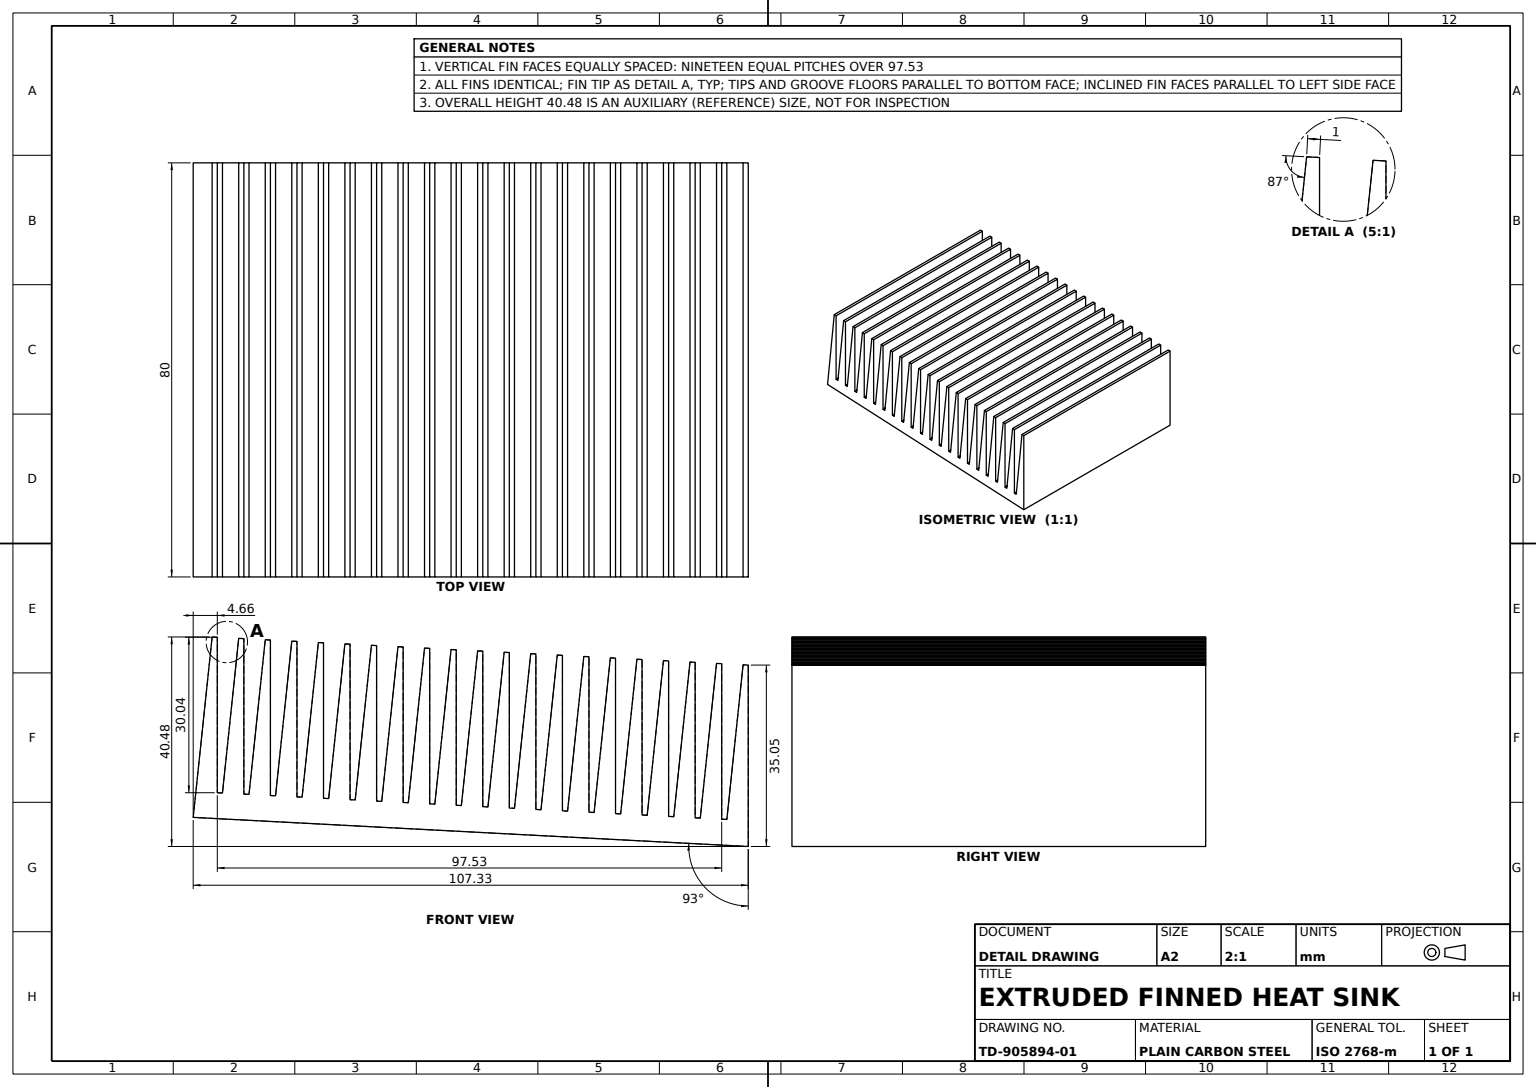
solid
v1 (-8.153019,80,-17.547966)
v2 (-6.580786,80,12.452034)
e1 v1 v2 LINE
v3 (-6.580786,0,12.452034)
e2 v2 v3 LINE
v4 (-8.153019,0,-17.547966)
e3 v4 v3 LINE
e4 v1 v4 LINE
face PLANE(AX(P(-7.213557,80,0.378046),D(0.998629535,0,-0.052335956),D(-0.052335956,0,-0.998629535))) [e1 e2 -e3 -e4]
v5 (-24.573019,80,-17.547966)
v6 (-24.573019,0,-17.547966)
e5 v5 v6 LINE
v7 (-26.145253,0,12.452034)
e6 v7 v6 LINE
v8 (-26.145253,80,12.452034)
e7 v8 v7 LINE
e8 v8 v5 LINE
face PLANE(AX(P(-25.422844,80,-1.332355),D(-0.998629535,0,-0.052335956),D(-0.052335956,0,0.998629535))) [e5 -e6 -e7 e8]
v9 (-11.720786,0,12.452034)
v10 (-10.725253,0,12.452034)
e9 v9 v10 LINE
v11 (-11.720786,80,12.452034)
e10 v11 v9 LINE
v12 (-10.725253,80,12.452034)
e11 v11 v12 LINE
e12 v12 v10 LINE
face PLANE(AX(P(0,80,12.452034),D(0,0,-1),D(-1,0,0))) [-e9 -e10 e11 e12]
v13 (1.126981,80,-17.547966)
v14 (2.126981,80,-17.547966)
e13 v13 v14 LINE
v15 (2.126981,0,-17.547966)
e14 v14 v15 LINE
v16 (1.126981,0,-17.547966)
e15 v16 v15 LINE
e16 v13 v16 LINE
face PLANE(AX(P(0,80,-17.547966),D(0,0,-1),D(-1,0,0))) [e13 e14 -e15 -e16]
v17 (-23.573019,0,-17.547966)
e17 v6 v17 LINE
v18 (-23.573019,80,-17.547966)
e18 v5 v18 LINE
e19 v18 v17 LINE
face PLANE(AX(P(0,80,-17.547966),D(0,0,-1),D(-1,0,0))) [-e17 -e5 e18 e19]
v19 (34.539214,80,12.452034)
v20 (34.539214,0,12.452034)
e20 v19 v20 LINE
v21 (32.966981,0,-17.547966)
e21 v21 v20 LINE
v22 (32.966981,80,-17.547966)
e22 v22 v21 LINE
e23 v22 v19 LINE
face PLANE(AX(P(33.793813,80,-1.771059),D(0.998629535,0,-0.052335956),D(-0.052335956,0,-0.998629535))) [e20 -e21 -e22 e23]
v23 (3.699214,80,12.452034)
v24 (3.699214,0,12.452034)
e24 v23 v24 LINE
v25 (4.694747,80,12.452034)
e25 v23 v25 LINE
v26 (4.694747,0,12.452034)
e26 v25 v26 LINE
e27 v24 v26 LINE
face PLANE(AX(P(0,80,12.452034),D(0,0,-1),D(-1,0,0))) [-e24 e25 e26 -e27]
v27 (48.386981,0,-17.547966)
v28 (49.959214,0,12.452034)
e28 v27 v28 LINE
v29 (48.386981,80,-17.547966)
e29 v29 v27 LINE
v30 (49.959214,80,12.452034)
e30 v29 v30 LINE
e31 v30 v28 LINE
face PLANE(AX(P(49.171577,80,-2.576973),D(0.998629535,0,-0.052335956),D(-0.052335956,0,-0.998629535))) [-e28 -e29 e30 e31]
v31 (50.954747,80,12.452034)
v32 (52.526981,80,-17.547966)
e32 v31 v32 LINE
v33 (52.526981,0,-17.547966)
e33 v32 v33 LINE
v34 (50.954747,0,12.452034)
e34 v34 v33 LINE
e35 v31 v34 LINE
face PLANE(AX(P(51.465975,80,2.697217),D(-0.998629535,0,-0.052335956),D(-0.052335956,0,0.998629535))) [e32 e33 -e34 -e35]
v35 (-16.860786,80,12.452034)
v36 (-15.865253,80,12.452034)
e36 v35 v36 LINE
v37 (-15.865253,0,12.452034)
e37 v36 v37 LINE
v38 (-16.860786,0,12.452034)
e38 v38 v37 LINE
e39 v35 v38 LINE
face PLANE(AX(P(0,80,12.452034),D(0,0,-1),D(-1,0,0))) [e36 e37 -e38 -e39]
v39 (40.674747,80,12.452034)
v40 (40.674747,0,12.452034)
e40 v39 v40 LINE
v41 (39.679214,0,12.452034)
e41 v41 v40 LINE
v42 (39.679214,80,12.452034)
e42 v42 v41 LINE
e43 v42 v39 LINE
face PLANE(AX(P(0,80,12.452034),D(0,0,-1),D(-1,0,0))) [e40 -e41 -e42 e43]
v43 (-5.585253,80,12.452034)
v44 (-5.585253,0,12.452034)
e44 v43 v44 LINE
e45 v3 v44 LINE
e46 v2 v43 LINE
face PLANE(AX(P(0,80,12.452034),D(0,0,-1),D(-1,0,0))) [e44 -e45 -e2 e46]
v45 (19.119214,0,12.452034)
v46 (20.114747,0,12.452034)
e47 v45 v46 LINE
v47 (19.119214,80,12.452034)
e48 v47 v45 LINE
v48 (20.114747,80,12.452034)
e49 v47 v48 LINE
e50 v48 v46 LINE
face PLANE(AX(P(0,80,12.452034),D(0,0,-1),D(-1,0,0))) [-e47 -e48 e49 e50]
v49 (8.839214,80,12.452034)
v50 (8.839214,0,12.452034)
e51 v49 v50 LINE
v51 (7.266981,0,-17.547966)
e52 v51 v50 LINE
v52 (7.266981,80,-17.547966)
e53 v52 v51 LINE
e54 v52 v49 LINE
face PLANE(AX(P(8.164207,80,-0.427868),D(0.998629535,0,-0.052335956),D(-0.052335956,0,-0.998629535))) [e51 -e52 -e53 e54]
v53 (-13.293019,80,-17.547966)
v54 (-13.293019,0,-17.547966)
e55 v53 v54 LINE
v55 (-14.293019,0,-17.547966)
e56 v55 v54 LINE
v56 (-14.293019,80,-17.547966)
e57 v56 v55 LINE
e58 v56 v53 LINE
face PLANE(AX(P(0,80,-17.547966),D(0,0,-1),D(-1,0,0))) [e55 -e56 -e57 e58]
v57 (56.094747,80,12.452034)
v58 (57.666981,80,-17.547966)
e59 v57 v58 LINE
v59 (57.666981,0,-17.547966)
e60 v58 v59 LINE
v60 (56.094747,0,12.452034)
e61 v60 v59 LINE
e62 v57 v60 LINE
face PLANE(AX(P(56.591897,80,2.965856),D(-0.998629535,0,-0.052335956),D(-0.052335956,0,0.998629535))) [e59 e60 -e61 -e62]
v61 (-32.280786,0,12.452034)
v62 (-31.285253,0,12.452034)
e63 v61 v62 LINE
v63 (-32.280786,80,12.452034)
e64 v63 v61 LINE
v64 (-31.285253,80,12.452034)
e65 v63 v64 LINE
e66 v64 v62 LINE
face PLANE(AX(P(0,80,12.452034),D(0,0,-1),D(-1,0,0))) [-e63 -e64 e65 e66]
e67 v54 v9 LINE
e68 v53 v11 LINE
face PLANE(AX(P(-12.339478,80,0.646685),D(0.998629535,0,-0.052335956),D(-0.052335956,0,-0.998629535))) [-e67 -e55 e68 e10]
v65 (53.526981,80,-17.547966)
v66 (53.526981,0,-17.547966)
e69 v65 v66 LINE
e70 v33 v66 LINE
e71 v32 v65 LINE
face PLANE(AX(P(0,80,-17.547966),D(0,0,-1),D(-1,0,0))) [e69 -e70 -e33 e71]
v67 (26.826981,80,-17.547966)
v68 (27.826981,80,-17.547966)
e72 v67 v68 LINE
v69 (27.826981,0,-17.547966)
e73 v68 v69 LINE
v70 (26.826981,0,-17.547966)
e74 v70 v69 LINE
e75 v67 v70 LINE
face PLANE(AX(P(0,80,-17.547966),D(0,0,-1),D(-1,0,0))) [e72 e73 -e74 -e75]
v71 (-9.153019,80,-17.547966)
e76 v71 v1 LINE
v72 (-9.153019,0,-17.547966)
e77 v72 v4 LINE
e78 v71 v72 LINE
face PLANE(AX(P(0,80,-17.547966),D(0,0,-1),D(-1,0,0))) [e76 e4 -e77 -e78]
v73 (-19.433019,80,-17.547966)
v74 (-19.433019,0,-17.547966)
e79 v73 v74 LINE
v75 (-18.433019,80,-17.547966)
e80 v73 v75 LINE
v76 (-18.433019,0,-17.547966)
e81 v75 v76 LINE
e82 v74 v76 LINE
face PLANE(AX(P(0,80,-17.547966),D(0,0,-1),D(-1,0,0))) [-e79 e80 e81 -e82]
v77 (-22.000786,80,12.452034)
e83 v18 v77 LINE
v78 (-22.000786,0,12.452034)
e84 v77 v78 LINE
e85 v17 v78 LINE
face PLANE(AX(P(-22.591321,80,1.183961),D(0.998629535,0,-0.052335956),D(-0.052335956,0,-0.998629535))) [e83 e84 -e85 -e19]
v79 (-37.425253,80,12.452034)
v80 (-36.425253,80,12.452034)
e86 v79 v80 LINE
v81 (-36.425253,0,12.452034)
e87 v80 v81 LINE
v82 (-37.425253,0,12.452034)
e88 v82 v81 LINE
e89 v79 v82 LINE
face PLANE(AX(P(0,80,12.452034),D(0,0,-1),D(-1,0,0))) [e86 e87 -e88 -e89]
v83 (9.834747,0,12.452034)
e90 v50 v83 LINE
v84 (9.834747,80,12.452034)
e91 v49 v84 LINE
e92 v84 v83 LINE
face PLANE(AX(P(0,80,12.452034),D(0,0,-1),D(-1,0,0))) [-e90 -e51 e91 e92]
v85 (61.234747,80,12.452034)
v86 (62.806981,80,-17.547966)
e93 v85 v86 LINE
v87 (62.806981,0,-17.547966)
e94 v86 v87 LINE
v88 (61.234747,0,12.452034)
e95 v88 v87 LINE
e96 v85 v88 LINE
face PLANE(AX(P(61.717818,80,3.234494),D(-0.998629535,0,-0.052335956),D(-0.052335956,0,0.998629535))) [e93 e94 -e95 -e96]
v89 (-38.997486,80,-17.547966)
v90 (-38.997486,0,-17.547966)
e97 v89 v90 LINE
e98 v89 v79 LINE
e99 v90 v82 LINE
face PLANE(AX(P(-37.973539,80,1.990109),D(0.998629535,0,-0.052335956),D(-0.052335956,0,-0.998629535))) [-e97 e98 e89 -e99]
v91 (-33.853019,0,-17.547966)
e100 v91 v61 LINE
v92 (-33.853019,80,-17.547966)
e101 v92 v91 LINE
e102 v92 v63 LINE
face PLANE(AX(P(-32.843163,80,1.721237),D(0.998629535,0,-0.052335956),D(-0.052335956,0,-0.998629535))) [e64 -e100 -e101 e102]
v93 (-34.853019,80,-17.547966)
e103 v93 v92 LINE
v94 (-34.853019,0,-17.547966)
e104 v94 v91 LINE
e105 v93 v94 LINE
face PLANE(AX(P(0,80,-17.547966),D(0,0,-1),D(-1,0,0))) [e103 e101 -e104 -e105]
v95 (24.259214,80,12.452034)
v96 (24.259214,0,12.452034)
e106 v95 v96 LINE
v97 (25.254747,80,12.452034)
e107 v95 v97 LINE
v98 (25.254747,0,12.452034)
e108 v97 v98 LINE
e109 v96 v98 LINE
face PLANE(AX(P(0,80,12.452034),D(0,0,-1),D(-1,0,0))) [-e106 e107 e108 -e109]
e110 v36 v56 LINE
e111 v37 v55 LINE
face PLANE(AX(P(-15.171001,80,-0.795078),D(-0.998629535,0,-0.052335956),D(-0.052335956,0,0.998629535))) [-e37 e110 e57 -e111]
v99 (14.974747,80,12.452034)
v100 (16.546981,80,-17.547966)
e112 v99 v100 LINE
v101 (16.546981,0,-17.547966)
e113 v100 v101 LINE
v102 (14.974747,0,12.452034)
e114 v102 v101 LINE
e115 v99 v102 LINE
face PLANE(AX(P(15.584527,80,0.81675),D(-0.998629535,0,-0.052335956),D(-0.052335956,0,0.998629535))) [e112 e113 -e114 -e115]
v103 (-21.005253,0,12.452034)
e116 v103 v74 LINE
v104 (-21.005253,80,12.452034)
e117 v104 v103 LINE
e118 v104 v73 LINE
face PLANE(AX(P(-20.296922,80,-1.063717),D(-0.998629535,0,-0.052335956),D(-0.052335956,0,0.998629535))) [-e116 -e117 e118 e79]
v105 (-39.997486,0,-17.547966)
e119 v105 v90 LINE
v106 (-39.997486,80,-17.547966)
e120 v106 v105 LINE
e121 v106 v89 LINE
face PLANE(AX(P(0,80,-17.547966),D(0,0,-1),D(-1,0,0))) [e97 -e119 -e120 e121]
v107 (-41.831758,80,17.452034)
v108 (65.641253,80,17.452034)
e122 v107 v108 LINE
v109 (-41.831758,0,17.452034)
e123 v107 v109 LINE
v110 (65.641253,0,17.452034)
e124 v109 v110 LINE
e125 v108 v110 LINE
face PLANE(AX(P(0,80,17.452034),D(0,0,-1),D(-1,0,0))) rev [-e122 e123 e124 -e125]
e126 v77 v104 LINE
e127 v78 v103 LINE
face PLANE(AX(P(0,80,12.452034),D(0,0,-1),D(-1,0,0))) [e126 e117 -e127 -e84]
v111 (42.246981,80,-17.547966)
v112 (43.246981,80,-17.547966)
e128 v111 v112 LINE
v113 (43.246981,0,-17.547966)
e129 v112 v113 LINE
v114 (42.246981,0,-17.547966)
e130 v114 v113 LINE
e131 v111 v114 LINE
face PLANE(AX(P(0,80,-17.547966),D(0,0,-1),D(-1,0,0))) [e128 e129 -e130 -e131]
v115 (6.266981,80,-17.547966)
e132 v115 v52 LINE
v116 (6.266981,0,-17.547966)
e133 v116 v51 LINE
e134 v115 v116 LINE
face PLANE(AX(P(0,80,-17.547966),D(0,0,-1),D(-1,0,0))) [e132 e53 -e133 -e134]
e135 v26 v116 LINE
e136 v25 v115 LINE
face PLANE(AX(P(5.332684,80,0.279474),D(-0.998629535,0,-0.052335956),D(-0.052335956,0,0.998629535))) [-e135 -e26 e136 e134]
v117 (21.686981,80,-17.547966)
v118 (21.686981,0,-17.547966)
e137 v117 v118 LINE
v119 (22.686981,80,-17.547966)
e138 v117 v119 LINE
v120 (22.686981,0,-17.547966)
e139 v119 v120 LINE
e140 v118 v120 LINE
face PLANE(AX(P(0,80,-17.547966),D(0,0,-1),D(-1,0,0))) [-e137 e138 e139 -e140]
v121 (30.394747,80,12.452034)
v122 (31.966981,80,-17.547966)
e141 v121 v122 LINE
v123 (31.966981,0,-17.547966)
e142 v122 v123 LINE
v124 (30.394747,0,12.452034)
e143 v124 v123 LINE
e144 v121 v124 LINE
face PLANE(AX(P(30.96229,80,1.622665),D(-0.998629535,0,-0.052335956),D(-0.052335956,0,0.998629535))) [e141 e142 -e143 -e144]
e145 v15 v24 LINE
e146 v14 v23 LINE
face PLANE(AX(P(3.038286,80,-0.15923),D(0.998629535,0,-0.052335956),D(-0.052335956,0,-0.998629535))) [e24 -e145 -e14 e146]
v125 (45.814747,80,12.452034)
v126 (45.814747,0,12.452034)
e147 v125 v126 LINE
v127 (44.819214,0,12.452034)
e148 v127 v126 LINE
v128 (44.819214,80,12.452034)
e149 v128 v127 LINE
e150 v128 v125 LINE
face PLANE(AX(P(0,80,12.452034),D(0,0,-1),D(-1,0,0))) [e147 -e148 -e149 e150]
v129 (-4.013019,80,-17.547966)
v130 (-3.013019,80,-17.547966)
e151 v129 v130 LINE
v131 (-3.013019,0,-17.547966)
e152 v130 v131 LINE
v132 (-4.013019,0,-17.547966)
e153 v132 v131 LINE
e154 v129 v132 LINE
face PLANE(AX(P(0,80,-17.547966),D(0,0,-1),D(-1,0,0))) [e151 e152 -e153 -e154]
v133 (63.806981,80,-17.547966)
v134 (63.806981,0,-17.547966)
e155 v133 v134 LINE
e156 v133 v108 LINE
e157 v134 v110 LINE
face PLANE(AX(P(64.549341,80,-3.382888),D(0.998629535,0,-0.052335956),D(-0.052335956,0,-0.998629535))) [-e155 e156 e125 -e157]
e158 v123 v21 LINE
e159 v122 v22 LINE
face PLANE(AX(P(0,80,-17.547966),D(0,0,-1),D(-1,0,0))) [-e158 -e142 e159 e22]
v135 (29.399214,80,12.452034)
v136 (29.399214,0,12.452034)
e160 v135 v136 LINE
e161 v69 v136 LINE
e162 v68 v135 LINE
face PLANE(AX(P(28.667892,80,-1.502421),D(0.998629535,0,-0.052335956),D(-0.052335956,0,-0.998629535))) [e160 -e161 -e73 e162]
e163 v44 v132 LINE
e164 v43 v129 LINE
face PLANE(AX(P(-4.919159,80,-0.257802),D(-0.998629535,0,-0.052335956),D(-0.052335956,0,0.998629535))) [-e163 -e44 e164 e154]
v137 (38.106981,0,-17.547966)
e165 v137 v41 LINE
v138 (38.106981,80,-17.547966)
e166 v138 v137 LINE
e167 v138 v42 LINE
face PLANE(AX(P(38.919735,80,-2.039697),D(0.998629535,0,-0.052335956),D(-0.052335956,0,-0.998629535))) [e42 -e165 -e166 e167]
v139 (-0.445253,0,12.452034)
e168 v139 v16 LINE
v140 (-0.445253,80,12.452034)
e169 v140 v139 LINE
e170 v140 v13 LINE
face PLANE(AX(P(0.206763,80,0.010836),D(-0.998629535,0,-0.052335956),D(-0.052335956,0,0.998629535))) [-e168 -e169 e170 e16]
v141 (11.406981,0,-17.547966)
e171 v83 v141 LINE
v142 (11.406981,80,-17.547966)
e172 v84 v142 LINE
e173 v142 v141 LINE
face PLANE(AX(P(10.458605,80,0.548112),D(-0.998629535,0,-0.052335956),D(-0.052335956,0,0.998629535))) [-e171 -e92 e172 e173]
e174 v87 v134 LINE
e175 v86 v133 LINE
face PLANE(AX(P(0,80,-17.547966),D(0,0,-1),D(-1,0,0))) [-e174 -e94 e175 e155]
e176 v30 v31 LINE
e177 v28 v34 LINE
face PLANE(AX(P(0,80,12.452034),D(0,0,-1),D(-1,0,0))) [-e31 e176 e35 -e177]
v143 (55.099214,0,12.452034)
e178 v143 v60 LINE
v144 (55.099214,80,12.452034)
e179 v144 v143 LINE
e180 v144 v57 LINE
face PLANE(AX(P(0,80,12.452034),D(0,0,-1),D(-1,0,0))) [-e178 -e179 e180 e62]
v145 (35.534747,0,12.452034)
v146 (37.106981,0,-17.547966)
e181 v145 v146 LINE
v147 (35.534747,80,12.452034)
e182 v147 v145 LINE
v148 (37.106981,80,-17.547966)
e183 v147 v148 LINE
e184 v148 v146 LINE
face PLANE(AX(P(36.088212,80,1.891303),D(-0.998629535,0,-0.052335956),D(-0.052335956,0,0.998629535))) [-e181 -e182 e183 e184]
e185 v120 v96 LINE
e186 v119 v95 LINE
face PLANE(AX(P(23.541971,80,-1.233782),D(0.998629535,0,-0.052335956),D(-0.052335956,0,-0.998629535))) [e106 -e185 -e139 e186]
v149 (-1.440786,80,12.452034)
e187 v130 v149 LINE
v150 (-1.440786,0,12.452034)
e188 v149 v150 LINE
e189 v131 v150 LINE
face PLANE(AX(P(-2.087636,80,0.109408),D(0.998629535,0,-0.052335956),D(-0.052335956,0,-0.998629535))) [-e152 e187 e188 -e189]
e190 v75 v35 LINE
v151 (-27.140786,80,12.452034)
e191 v151 v8 LINE
v152 (-28.713019,80,-17.547966)
e192 v152 v151 LINE
v153 (-29.713019,80,-17.547966)
e193 v153 v152 LINE
e194 v64 v153 LINE
e195 v80 v93 LINE
e196 v106 v107 LINE
v154 (60.239214,80,12.452034)
e197 v154 v85 LINE
v155 (58.666981,80,-17.547966)
e198 v155 v154 LINE
e199 v58 v155 LINE
e200 v65 v144 LINE
v156 (47.386981,80,-17.547966)
e201 v156 v29 LINE
e202 v125 v156 LINE
e203 v112 v128 LINE
e204 v39 v111 LINE
e205 v148 v138 LINE
e206 v19 v147 LINE
e207 v135 v121 LINE
e208 v97 v67 LINE
e209 v48 v117 LINE
v157 (17.546981,80,-17.547966)
e210 v157 v47 LINE
e211 v100 v157 LINE
v158 (13.979214,80,12.452034)
e212 v158 v99 LINE
v159 (12.406981,80,-17.547966)
e213 v159 v158 LINE
e214 v142 v159 LINE
e215 v149 v140 LINE
e216 v12 v71 LINE
face PLANE(AX(P(0,80,0),D(0,1,0),D(0,0,1))) [-e36 -e190 -e80 -e118 -e126 -e83 -e18 -e8 -e191 -e192 -e193 -e194 -e65 -e102 -e103 -e195 -e86 -e98 -e121 e196 e122 -e156 -e175 -e93 -e197 -e198 -e199 -e59 -e180 -e200 -e71 -e32 -e176 -e30 -e201 -e202 -e150 -e203 -e128 -e204 -e43 -e167 -e205 -e183 -e206 -e23 -e159 -e141 -e207 -e162 -e72 -e208 -e107 -e186 -e138 -e209 -e49 -e210 -e211 -e112 -e212 -e213 -e214 -e172 -e91 -e54 -e132 -e136 -e25 -e146 -e13 -e170 -e215 -e187 -e151 -e164 -e46 -e1 -e76 -e216 -e11 -e68 -e58 -e110]
v160 (-29.713019,0,-17.547966)
e217 v62 v160 LINE
e218 v153 v160 LINE
face PLANE(AX(P(-30.548765,80,-1.600993),D(-0.998629535,0,-0.052335956),D(-0.052335956,0,0.998629535))) [-e217 -e66 e194 e218]
e219 v20 v145 LINE
face PLANE(AX(P(0,80,12.452034),D(0,0,-1),D(-1,0,0))) [-e219 -e20 e206 e182]
e220 v66 v143 LINE
face PLANE(AX(P(54.297498,80,-2.845611),D(0.998629535,0,-0.052335956),D(-0.052335956,0,-0.998629535))) [e200 e179 -e220 -e69]
v161 (60.239214,0,12.452034)
e221 v161 v88 LINE
e222 v154 v161 LINE
face PLANE(AX(P(0,80,12.452034),D(0,0,-1),D(-1,0,0))) [-e221 -e222 e197 e96]
e223 v10 v72 LINE
face PLANE(AX(P(-10.04508,80,-0.52644),D(-0.998629535,0,-0.052335956),D(-0.052335956,0,0.998629535))) [e78 -e223 -e12 e216]
e224 v76 v38 LINE
face PLANE(AX(P(-17.465399,80,0.915323),D(0.998629535,0,-0.052335956),D(-0.052335956,0,-0.998629535))) [-e81 e190 e39 -e224]
e225 v150 v139 LINE
face PLANE(AX(P(0,80,12.452034),D(0,0,-1),D(-1,0,0))) [-e188 e215 e169 -e225]
v162 (58.666981,0,-17.547966)
e226 v155 v162 LINE
e227 v162 v161 LINE
face PLANE(AX(P(59.42342,80,-3.114249),D(0.998629535,0,-0.052335956),D(-0.052335956,0,-0.998629535))) [-e226 e198 e222 -e227]
e228 v146 v137 LINE
face PLANE(AX(P(0,80,-17.547966),D(0,0,-1),D(-1,0,0))) [-e228 -e184 e205 e166]
v163 (47.386981,0,-17.547966)
e229 v156 v163 LINE
e230 v126 v163 LINE
face PLANE(AX(P(46.340054,80,2.428579),D(-0.998629535,0,-0.052335956),D(-0.052335956,0,0.998629535))) [-e147 e202 e229 -e230]
e231 v59 v162 LINE
face PLANE(AX(P(0,80,-17.547966),D(0,0,-1),D(-1,0,0))) [-e60 e199 e226 -e231]
v164 (-27.140786,0,12.452034)
e232 v151 v164 LINE
v165 (-28.713019,0,-17.547966)
e233 v165 v164 LINE
e234 v152 v165 LINE
face PLANE(AX(P(-27.717242,80,1.452599),D(0.998629535,0,-0.052335956),D(-0.052335956,0,-0.998629535))) [e192 e232 -e233 -e234]
e235 v40 v114 LINE
face PLANE(AX(P(41.214133,80,2.159941),D(-0.998629535,0,-0.052335956),D(-0.052335956,0,0.998629535))) [-e40 e204 e131 -e235]
v166 (12.406981,0,-17.547966)
e236 v159 v166 LINE
e237 v141 v166 LINE
face PLANE(AX(P(0,80,-17.547966),D(0,0,-1),D(-1,0,0))) [e236 -e237 -e173 e214]
v167 (13.979214,0,12.452034)
e238 v167 v102 LINE
e239 v158 v167 LINE
face PLANE(AX(P(0,80,12.452034),D(0,0,-1),D(-1,0,0))) [-e238 -e239 e212 e115]
e240 v81 v94 LINE
face PLANE(AX(P(-35.674686,80,-1.869631),D(-0.998629535,0,-0.052335956),D(-0.052335956,0,0.998629535))) [e195 e105 -e240 -e87]
e241 v166 v167 LINE
face PLANE(AX(P(13.290128,80,-0.696506),D(0.998629535,0,-0.052335956),D(-0.052335956,0,-0.998629535))) [-e241 -e236 e213 e239]
v168 (17.546981,0,-17.547966)
e242 v168 v45 LINE
e243 v157 v168 LINE
face PLANE(AX(P(18.416049,80,-0.965144),D(0.998629535,0,-0.052335956),D(-0.052335956,0,-0.998629535))) [e48 -e242 -e243 e210]
e244 v105 v109 LINE
face PLANE(AX(P(-40.805062,80,-2.138503),D(0.998629535,0,0.052335956),D(0.052335956,0,-0.998629535))) rev [-e196 e120 e244 -e123]
e245 v160 v165 LINE
face PLANE(AX(P(0,80,-17.547966),D(0,0,-1),D(-1,0,0))) [e193 e234 -e245 -e218]
e246 v113 v127 LINE
face PLANE(AX(P(44.045656,80,-2.308335),D(0.998629535,0,-0.052335956),D(-0.052335956,0,-0.998629535))) [e203 e149 -e246 -e129]
e247 v163 v27 LINE
face PLANE(AX(P(0,80,-17.547966),D(0,0,-1),D(-1,0,0))) [-e247 -e229 e201 e29]
e248 v164 v7 LINE
face PLANE(AX(P(0,80,12.452034),D(0,0,-1),D(-1,0,0))) [e7 -e248 -e232 e191]
e249 v101 v168 LINE
face PLANE(AX(P(0,80,-17.547966),D(0,0,-1),D(-1,0,0))) [e243 -e249 -e113 e211]
e250 v46 v118 LINE
face PLANE(AX(P(20.710448,80,1.085389),D(-0.998629535,0,-0.052335956),D(-0.052335956,0,0.998629535))) [e137 -e250 -e50 e209]
e251 v98 v70 LINE
e252 v136 v124 LINE
face PLANE(AX(P(0,0,0),D(0,1,0),D(0,0,1))) rev [e163 e153 e189 e225 e168 e15 e145 e27 e135 e133 e52 e90 e171 e237 e241 e238 e114 e249 e242 e47 e250 e140 e185 e109 e251 e74 e161 e252 e143 e158 e21 e219 e181 e228 e165 e41 e235 e130 e246 e148 e230 e247 e28 e177 e34 e70 e220 e178 e61 e231 e227 e221 e95 e174 e157 -e124 -e244 e119 e99 e88 e240 e104 e100 e63 e217 e245 e233 e248 e6 e17 e85 e127 e116 e82 e224 e38 e111 e56 e67 e9 e223 e77 e3 e45]
face PLANE(AX(P(25.836369,80,1.354027),D(-0.998629535,0,-0.052335956),D(-0.052335956,0,0.998629535))) [-e251 -e108 e208 e75]
face PLANE(AX(P(0,80,12.452034),D(0,0,-1),D(-1,0,0))) [e207 e144 -e252 -e160]
